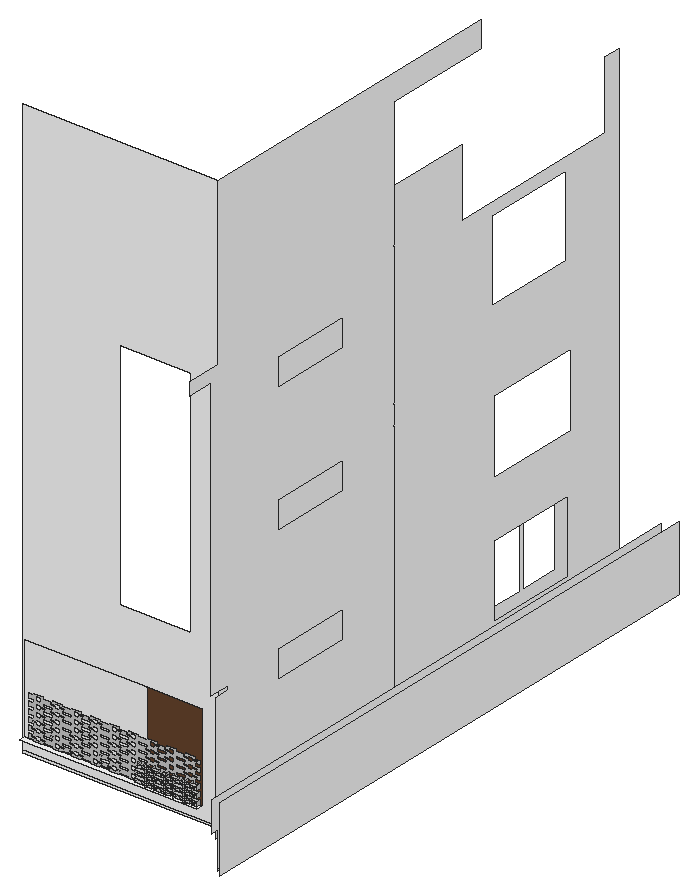
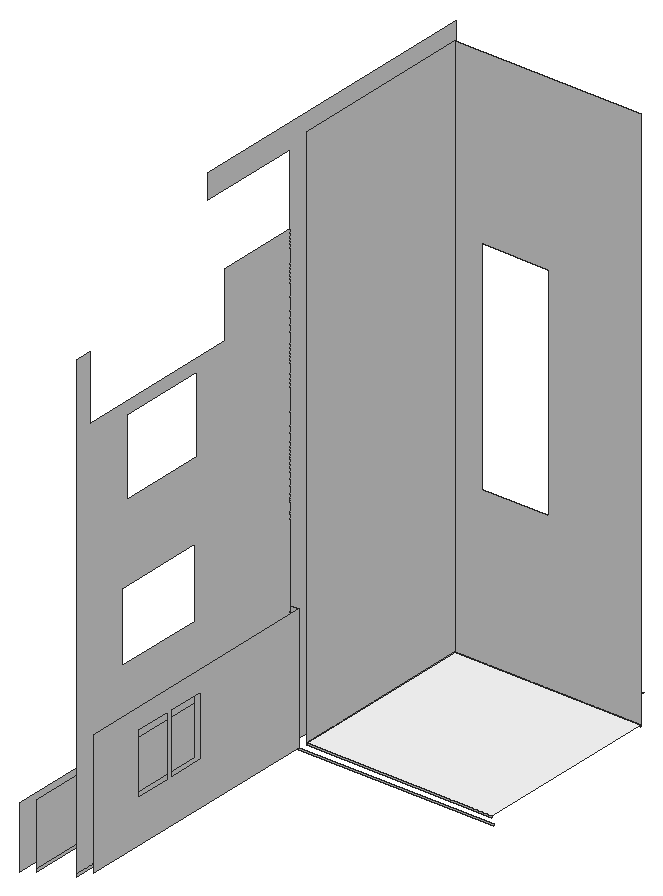
# SketchUp Ruby script. Lengths in inches.
U = 1.inch
M = Sketchup.active_model
def pt(a) = Geom::Point3d.new(a.map { |v| v * U })
def face(e, loops, mat)
  f = e.add_face(loops[0].map { |a| pt(a) })
  loops[1..].each { |l| e.add_face(l.map { |a| pt(a) }).erase! }
  f.material = f.back_material = mat if mat
  f
end
# faces: each face lists its corners as indices into pts; further lists are holes
def faces(e, pts, list, mat = nil) = list.each { |f| face(e, (f[0].is_a?(Array) ? f : [f]).map { |l| l.map { |i| pts[i] } }, mat) }
# xy, xz, yz: faces in a plane at the given z, y or x. An outline is a flat list of corners, or four numbers for a rectangle; further outlines are holes
def ring(l) = l.size == 4 ? [[l[0], l[1]], [l[2], l[1]], [l[2], l[3]], [l[0], l[3]]] : l.each_slice(2).to_a
def flat(e, list, mat, &to3) = list.each { |f| face(e, (f[0].is_a?(Array) ? f : [f]).map { |l| ring(l).map { |u, v| to3.(u, v) } }, mat) }
def xy(e, z, list, mat = nil) = flat(e, list, mat) { |x, y| [x, y, z] }
def xz(e, y, list, mat = nil) = flat(e, list, mat) { |x, z| [x, y, z] }
def yz(e, x, list, mat = nil) = flat(e, list, mat) { |y, z| [x, y, z] }
def lines(e, pts, list) = list.each { |a, b| e.add_line(pt(pts[a]), pt(pts[b])) }
# prism: a flat outline (further loops are holes) pulled along v
def prism(e, loops, v, mat = nil)
  f = face(e, loops, mat); d = Geom::Vector3d.new(v.map { |x| x * U })
  f.pushpull(f.normal.samedirection?(d) ? d.length : -d.length)
end
def box(e, o, s, mat = nil) = prism(e, [[o, [o[0] + s[0], o[1], o[2]], [o[0] + s[0], o[1] + s[1], o[2]], [o[0], o[1] + s[1], o[2]]]], [0, 0, s[2]], mat)
def at(x, y, z, deg = 0) = Geom::Transformation.translation(pt([x, y, z])) * Geom::Transformation.rotation(ORIGIN, Z_AXIS, deg.degrees)
def axes(o, x, y, z) = Geom::Transformation.new([*x, 0, *y, 0, *z, 0, *pt(o).to_a, 1])
def part(name) = M.definitions.add(name)
# library, detail: a bought-in or finely detailed component or shape, given as its bounding box
def library(name, o, s) = part(name).tap { |d| box(d.entities, o, s) }
def detail(e, o, s) = box(e.add_group.entities, o, s)
def put(e, d, t, mat = nil) = e.add_instance(d, t).tap { |i| i.material = mat if mat }
def group(e, t, mat = nil) = e.add_group.tap { |g| g.transformation = t; g.material = mat if mat }.entities
root = M.entities
M.materials.add("M00_Soft_Cloud").color = [255, 255, 255]
M.materials.add("Metal_Perforated_03_1K").color = [205, 205, 205]
M.materials.add("Wood_Veneer_15_1K1").color = [103, 69, 45]
xy(root,0,[[375,129,555,309]],"M00_Soft_Cloud")
xy(root,18,[[384,114,546,120]],"M00_Soft_Cloud")
xy(root,18,[[497.5,115.4375,505.72,119.17],[514.95,115.4375,523.18,119.17],[532.4,115.4375,540.63,119.17]],"Metal_Perforated_03_1K")
xy(root,19.23,[[499.55,115.4375,503.68,119.17],[517,115.4375,521.13,119.17],[534.45,115.4375,538.58,119.17]],"Metal_Perforated_03_1K")
xy(root,19.33,[[488.27,115.4375,497.5,119.17],[505.72,115.4375,514.95,119.17],[523.18,115.4375,532.4,119.17],[540.63,115.4375,545.24,119.17]],"Metal_Perforated_03_1K")
xy(root,20.57,[[494.94,115.4375,499.55,119.17],[503.68,115.4375,508.29,119.17],[512.39,115.4375,517,119.17],[521.13,115.4375,525.74,119.17],[529.84,115.4375,534.45,119.17],
  [538.58,115.4375,543.19,119.17]],"Metal_Perforated_03_1K")
xy(root,21.93,[[494.94,115.4375,499.55,119.17],[503.68,115.4375,508.29,119.17],[512.39,115.4375,517,119.17],[521.13,115.4375,525.74,119.17],[529.84,115.4375,534.45,119.17],
  [538.58,115.4375,543.19,119.17]],"Metal_Perforated_03_1K")
xy(root,23.16,[[488.27,115.4375,497.5,119.17],[505.72,115.4375,514.95,119.17],[523.18,115.4375,532.4,119.17],[540.63,115.4375,545.24,119.17]],"Metal_Perforated_03_1K")
xy(root,23.26,[[499.55,115.4375,503.68,119.17],[517,115.4375,521.13,119.17],[534.45,115.4375,538.58,119.17]],"Metal_Perforated_03_1K")
xy(root,25.73,[[499.55,115.4375,503.68,119.17],[517,115.4375,521.13,119.17],[534.45,115.4375,538.58,119.17]],"Metal_Perforated_03_1K")
xy(root,25.83,[[488.27,115.4375,497.5,119.17],[505.72,115.4375,514.95,119.17],[523.18,115.4375,532.4,119.17],[540.63,115.4375,545.24,119.17]],"Metal_Perforated_03_1K")
xy(root,27.06,[[494.94,115.4375,499.55,119.17],[503.68,115.4375,508.29,119.17],[512.39,115.4375,517,119.17],[521.13,115.4375,525.74,119.17],[529.84,115.4375,534.45,119.17],
  [538.58,115.4375,543.19,119.17]],"Metal_Perforated_03_1K")
xy(root,28.42,[[494.94,115.4375,499.55,119.17],[503.68,115.4375,508.29,119.17],[512.39,115.4375,517,119.17],[521.13,115.4375,525.74,119.17],[529.84,115.4375,534.45,119.17],
  [538.58,115.4375,543.19,119.17]],"Metal_Perforated_03_1K")
xy(root,29.65,[[488.27,115.4375,497.5,119.17],[505.72,115.4375,514.95,119.17],[523.18,115.4375,532.4,119.17],[540.63,115.4375,545.24,119.17]],"Metal_Perforated_03_1K")
xy(root,29.75,[[499.55,115.4375,503.68,119.17],[517,115.4375,521.13,119.17],[534.45,115.4375,538.58,119.17]],"Metal_Perforated_03_1K")
xy(root,32.22,[[499.55,115.4375,503.68,119.17],[517,115.4375,521.13,119.17],[534.45,115.4375,538.58,119.17]],"Metal_Perforated_03_1K")
xy(root,32.32,[[488.27,115.4375,497.5,119.17],[505.72,115.4375,514.95,119.17],[523.18,115.4375,532.4,119.17],[540.63,115.4375,545.24,119.17]],"Metal_Perforated_03_1K")
xy(root,33.55,[[494.94,115.4375,499.55,119.17],[503.68,115.4375,508.29,119.17],[512.39,115.4375,517,119.17],[521.13,115.4375,525.74,119.17],[529.84,115.4375,534.45,119.17],
  [538.58,115.4375,543.19,119.17]],"Metal_Perforated_03_1K")
xy(root,34.91,[[494.94,115.4375,499.55,119.17],[503.68,115.4375,508.29,119.17],[512.39,115.4375,517,119.17],[521.13,115.4375,525.74,119.17],[529.84,115.4375,534.45,119.17],
  [538.58,115.4375,543.19,119.17]],"Metal_Perforated_03_1K")
xz(root,119.17,[[[392.79,18,401.01,18,401.01,19.33,410.24,19.33,410.24,18,418.47,18,418.47,19.33,427.69,19.33,427.69,18,435.92,18,435.92,19.33,445.15,19.33,445.15,18,453.37,18,453.37,19.33,462.6,19.33,462.6,18,470.82,18,470.82,19.33,480.05,19.33,480.05,18,488.27,18,488.27,19.33,497.5,19.33,497.5,18,505.72,18,505.72,19.33,514.95,19.33,514.95,18,523.18,18,523.18,19.33,532.4,19.33,532.4,18,540.63,18,540.63,19.33,545.24,19.33,545.24,23.16,540.63,23.16,540.63,25.83,545.24,25.83,545.24,29.65,540.63,29.65,540.63,32.32,545.24,32.32,545.24,36.14,540.63,36.14,540.63,38.8125,545.24,38.8125,545.24,42.64,540.63,42.64,540.63,45.31,545.24,45.31,545.24,49.13,540.63,49.13,540.63,51.8,545.24,51.8,545.24,55.62,540.63,55.62,540.63,56.96,532.4,56.96,532.4,55.62,523.18,55.62,523.18,56.96,514.95,56.96,514.95,55.62,505.72,55.62,505.72,56.96,497.5,56.96,497.5,55.62,488.27,55.62,488.27,56.96,480.05,56.96,480.05,55.62,470.82,55.62,470.82,56.96,462.6,56.96,462.6,55.62,453.37,55.62,453.37,56.96,445.15,56.96,445.15,55.62,435.92,55.62,435.92,56.96,427.69,56.96,427.69,55.62,418.47,55.62,418.47,56.96,410.24,56.96,410.24,55.62,401.01,55.62,401.01,56.96,392.79,56.96,392.79,55.62,388.18,55.62,388.18,51.8,392.79,51.8,392.79,49.13,388.18,49.13,388.18,45.31,392.79,45.31,392.79,42.64,388.18,42.64,388.18,38.8125,392.79,38.8125,392.79,36.14,388.18,36.14,388.18,32.32,392.79,32.32,392.79,29.65,388.18,29.65,388.18,25.83,392.79,25.83,392.79,23.16,388.18,23.16,388.18,19.33,392.79,19.33],[464.65,51.7,464.65,53.03,460.03,53.03,460.03,54.39,464.65,54.39,464.65,55.72,468.77,55.72,468.77,54.39,473.39,54.39,473.39,53.03,468.77,53.03,468.77,51.7],[482.1,51.7,482.1,53.03,477.48,53.03,477.48,54.39,482.1,54.39,482.1,55.72,486.22,55.72,486.22,54.39,490.84,54.39,490.84,53.03,486.22,53.03,486.22,51.7],[464.65,25.73,464.65,27.06,460.03,27.06,460.03,28.42,464.65,28.42,464.65,29.75,468.77,29.75,468.77,28.42,473.39,28.42,473.39,27.06,468.77,27.06,468.77,25.73],[464.65,32.22,464.65,33.55,460.03,33.55,460.03,34.91,464.65,34.91,464.65,36.25,468.77,36.25,468.77,34.91,473.39,34.91,473.39,33.55,468.77,33.55,468.77,32.22],[464.65,19.23,464.65,20.57,460.03,20.57,460.03,21.93,464.65,21.93,464.65,23.26,468.77,23.26,468.77,21.93,473.39,21.93,473.39,20.57,468.77,20.57,468.77,19.23],[464.65,45.2,464.65,46.54,460.03,46.54,460.03,47.9,464.65,47.9,464.65,49.23,468.77,49.23,468.77,47.9,473.39,47.9,473.39,46.54,468.77,46.54,468.77,45.2],[482.1,25.73,482.1,27.06,477.48,27.06,477.48,28.42,482.1,28.42,482.1,29.75,486.22,29.75,486.22,28.42,490.84,28.42,490.84,27.06,486.22,27.06,486.22,25.73],[482.1,32.22,482.1,33.55,477.48,33.55,477.48,34.91,482.1,34.91,482.1,36.25,486.22,36.25,486.22,34.91,490.84,34.91,490.84,33.55,486.22,33.55,486.22,32.22],[482.1,19.23,482.1,20.57,477.48,20.57,477.48,21.93,482.1,21.93,482.1,23.26,486.22,23.26,486.22,21.93,490.84,21.93,490.84,20.57,486.22,20.57,486.22,19.23],[482.1,45.2,482.1,46.54,477.48,46.54,477.48,47.9,482.1,47.9,482.1,49.23,486.22,49.23,486.22,47.9,490.84,47.9,490.84,46.54,486.22,46.54,486.22,45.2],[464.65,38.71,464.65,40.05,460.03,40.05,460.03,41.4,464.65,41.4,464.65,42.74,468.77,42.74,468.77,41.4,473.39,41.4,473.39,40.05,468.77,40.05,468.77,38.71],[482.1,38.71,482.1,40.05,477.48,40.05,477.48,41.4,482.1,41.4,482.1,42.74,486.22,42.74,486.22,41.4,490.84,41.4,490.84,40.05,486.22,40.05,486.22,38.71],[394.84,51.7,394.84,53.03,390.22,53.03,390.22,54.39,394.84,54.39,394.84,55.72,398.97,55.72,398.97,54.39,403.58,54.39,403.58,53.03,398.97,53.03,398.97,51.7],[394.84,25.73,394.84,27.06,390.22,27.06,390.22,28.42,394.84,28.42,394.84,29.75,398.97,29.75,398.97,28.42,403.58,28.42,403.58,27.06,398.97,27.06,398.97,25.73],[394.84,19.23,394.84,20.57,390.22,20.57,390.22,21.93,394.84,21.93,394.84,23.26,398.97,23.26,398.97,21.93,403.58,21.93,403.58,20.57,398.97,20.57,398.97,19.23],[394.84,32.22,394.84,33.55,390.22,33.55,390.22,34.91,394.84,34.91,394.84,36.25,398.97,36.25,398.97,34.91,403.58,34.91,403.58,33.55,398.97,33.55,398.97,32.22],[394.84,45.2,394.84,46.54,390.22,46.54,390.22,47.9,394.84,47.9,394.84,49.23,398.97,49.23,398.97,47.9,403.58,47.9,403.58,46.54,398.97,46.54,398.97,45.2],[517,51.7,517,53.03,512.39,53.03,512.39,54.39,517,54.39,517,55.72,521.13,55.72,521.13,54.39,525.74,54.39,525.74,53.03,521.13,53.03,521.13,51.7],[517,25.73,517,27.06,512.39,27.06,512.39,28.42,517,28.42,517,29.75,521.13,29.75,521.13,28.42,525.74,28.42,525.74,27.06,521.13,27.06,521.13,25.73],[517,32.22,517,33.55,512.39,33.55,512.39,34.91,517,34.91,517,36.25,521.13,36.25,521.13,34.91,525.74,34.91,525.74,33.55,521.13,33.55,521.13,32.22],[517,19.23,517,20.57,512.39,20.57,512.39,21.93,517,21.93,517,23.26,521.13,23.26,521.13,21.93,525.74,21.93,525.74,20.57,521.13,20.57,521.13,19.23],[394.84,38.71,394.84,40.05,390.22,40.05,390.22,41.4,394.84,41.4,394.84,42.74,398.97,42.74,398.97,41.4,403.58,41.4,403.58,40.05,398.97,40.05,398.97,38.71],[517,45.2,517,46.54,512.39,46.54,512.39,47.9,517,47.9,517,49.23,521.13,49.23,521.13,47.9,525.74,47.9,525.74,46.54,521.13,46.54,521.13,45.2],[517,38.71,517,40.05,512.39,40.05,512.39,41.4,517,41.4,517,42.74,521.13,42.74,521.13,41.4,525.74,41.4,525.74,40.05,521.13,40.05,521.13,38.71],[412.29,51.7,412.29,53.03,407.68,53.03,407.68,54.39,412.29,54.39,412.29,55.72,416.42,55.72,416.42,54.39,421.03,54.39,421.03,53.03,416.42,53.03,416.42,51.7],[412.29,19.23,412.29,20.57,407.68,20.57,407.68,21.93,412.29,21.93,412.29,23.26,416.42,23.26,416.42,21.93,421.03,21.93,421.03,20.57,416.42,20.57,416.42,19.23],[429.74,51.7,429.74,53.03,425.13,53.03,425.13,54.39,429.74,54.39,429.74,55.72,433.87,55.72,433.87,54.39,438.48,54.39,438.48,53.03,433.87,53.03,433.87,51.7],[412.29,25.73,412.29,27.06,407.68,27.06,407.68,28.42,412.29,28.42,412.29,29.75,416.42,29.75,416.42,28.42,421.03,28.42,421.03,27.06,416.42,27.06,416.42,25.73],[412.29,32.22,412.29,33.55,407.68,33.55,407.68,34.91,412.29,34.91,412.29,36.25,416.42,36.25,416.42,34.91,421.03,34.91,421.03,33.55,416.42,33.55,416.42,32.22],[412.29,45.2,412.29,46.54,407.68,46.54,407.68,47.9,412.29,47.9,412.29,49.23,416.42,49.23,416.42,47.9,421.03,47.9,421.03,46.54,416.42,46.54,416.42,45.2],[429.74,32.22,429.74,33.55,425.13,33.55,425.13,34.91,429.74,34.91,429.74,36.25,433.87,36.25,433.87,34.91,438.48,34.91,438.48,33.55,433.87,33.55,433.87,32.22],[429.74,25.73,429.74,27.06,425.13,27.06,425.13,28.42,429.74,28.42,429.74,29.75,433.87,29.75,433.87,28.42,438.48,28.42,438.48,27.06,433.87,27.06,433.87,25.73],[429.74,19.23,429.74,20.57,425.13,20.57,425.13,21.93,429.74,21.93,429.74,23.26,433.87,23.26,433.87,21.93,438.48,21.93,438.48,20.57,433.87,20.57,433.87,19.23],[429.74,45.2,429.74,46.54,425.13,46.54,425.13,47.9,429.74,47.9,429.74,49.23,433.87,49.23,433.87,47.9,438.48,47.9,438.48,46.54,433.87,46.54,433.87,45.2],[534.45,51.7,534.45,53.03,529.84,53.03,529.84,54.39,534.45,54.39,534.45,55.72,538.58,55.72,538.58,54.39,543.19,54.39,543.19,53.03,538.58,53.03,538.58,51.7],[412.29,38.71,412.29,40.05,407.68,40.05,407.68,41.4,412.29,41.4,412.29,42.74,416.42,42.74,416.42,41.4,421.03,41.4,421.03,40.05,416.42,40.05,416.42,38.71],[534.45,25.73,534.45,27.06,529.84,27.06,529.84,28.42,534.45,28.42,534.45,29.75,538.58,29.75,538.58,28.42,543.19,28.42,543.19,27.06,538.58,27.06,538.58,25.73],[447.19,51.7,447.19,53.03,442.58,53.03,442.58,54.39,447.19,54.39,447.19,55.72,451.32,55.72,451.32,54.39,455.93,54.39,455.93,53.03,451.32,53.03,451.32,51.7],[534.45,32.22,534.45,33.55,529.84,33.55,529.84,34.91,534.45,34.91,534.45,36.25,538.58,36.25,538.58,34.91,543.19,34.91,543.19,33.55,538.58,33.55,538.58,32.22],[534.45,19.23,534.45,20.57,529.84,20.57,529.84,21.93,534.45,21.93,534.45,23.26,538.58,23.26,538.58,21.93,543.19,21.93,543.19,20.57,538.58,20.57,538.58,19.23],[429.74,38.71,429.74,40.05,425.13,40.05,425.13,41.4,429.74,41.4,429.74,42.74,433.87,42.74,433.87,41.4,438.48,41.4,438.48,40.05,433.87,40.05,433.87,38.71],[534.45,45.2,534.45,46.54,529.84,46.54,529.84,47.9,534.45,47.9,534.45,49.23,538.58,49.23,538.58,47.9,543.19,47.9,543.19,46.54,538.58,46.54,538.58,45.2],[447.19,25.73,447.19,27.06,442.58,27.06,442.58,28.42,447.19,28.42,447.19,29.75,451.32,29.75,451.32,28.42,455.93,28.42,455.93,27.06,451.32,27.06,451.32,25.73],[447.19,19.23,447.19,20.57,442.58,20.57,442.58,21.93,447.19,21.93,447.19,23.26,451.32,23.26,451.32,21.93,455.93,21.93,455.93,20.57,451.32,20.57,451.32,19.23],[447.19,32.22,447.19,33.55,442.58,33.55,442.58,34.91,447.19,34.91,447.19,36.25,451.32,36.25,451.32,34.91,455.93,34.91,455.93,33.55,451.32,33.55,451.32,32.22],[447.19,45.2,447.19,46.54,442.58,46.54,442.58,47.9,447.19,47.9,447.19,49.23,451.32,49.23,451.32,47.9,455.93,47.9,455.93,46.54,451.32,46.54,451.32,45.2],[534.45,38.71,534.45,40.05,529.84,40.05,529.84,41.4,534.45,41.4,534.45,42.74,538.58,42.74,538.58,41.4,543.19,41.4,543.19,40.05,538.58,40.05,538.58,38.71],[499.55,51.7,499.55,53.03,494.94,53.03,494.94,54.39,499.55,54.39,499.55,55.72,503.68,55.72,503.68,54.39,508.29,54.39,508.29,53.03,503.68,53.03,503.68,51.7],[447.19,38.71,447.19,40.05,442.58,40.05,442.58,41.4,447.19,41.4,447.19,42.74,451.32,42.74,451.32,41.4,455.93,41.4,455.93,40.05,451.32,40.05,451.32,38.71],[499.55,25.73,499.55,27.06,494.94,27.06,494.94,28.42,499.55,28.42,499.55,29.75,503.68,29.75,503.68,28.42,508.29,28.42,508.29,27.06,503.68,27.06,503.68,25.73],[499.55,19.23,499.55,20.57,494.94,20.57,494.94,21.93,499.55,21.93,499.55,23.26,503.68,23.26,503.68,21.93,508.29,21.93,508.29,20.57,503.68,20.57,503.68,19.23],[499.55,32.22,499.55,33.55,494.94,33.55,494.94,34.91,499.55,34.91,499.55,36.25,503.68,36.25,503.68,34.91,508.29,34.91,508.29,33.55,503.68,33.55,503.68,32.22],[499.55,45.2,499.55,46.54,494.94,46.54,494.94,47.9,499.55,47.9,499.55,49.23,503.68,49.23,503.68,47.9,508.29,47.9,508.29,46.54,503.68,46.54,503.68,45.2],[499.55,38.71,499.55,40.05,494.94,40.05,494.94,41.4,499.55,41.4,499.55,42.74,503.68,42.74,503.68,41.4,508.29,41.4,508.29,40.05,503.68,40.05,503.68,38.71],[418.47,36.14,427.69,38.8125],[470.82,36.14,480.05,38.8125],[418.47,42.64,427.69,45.31],[418.47,29.65,427.69,32.32],[470.82,42.64,480.05,45.31],[470.82,29.65,480.05,32.32],[418.47,23.16,427.69,25.83],[470.82,23.16,480.05,25.83],[418.47,49.13,427.69,51.8],[470.82,49.13,480.05,51.8],[488.27,36.14,497.5,38.8125],[488.27,42.64,497.5,45.31],[488.27,29.65,497.5,32.32],[488.27,23.16,497.5,25.83],[488.27,49.13,497.5,51.8],[453.37,36.14,462.6,38.8125],[453.37,29.65,462.6,32.32],[523.18,36.14,532.4,38.8125],[453.37,23.16,462.6,25.83],[523.18,42.64,532.4,45.31],[453.37,42.64,462.6,45.31],[523.18,29.65,532.4,32.32],[523.18,23.16,532.4,25.83],[453.37,49.13,462.6,51.8],[505.72,36.14,514.95,38.8125],[435.92,36.14,445.15,38.8125],[435.92,42.64,445.15,45.31],[523.18,49.13,532.4,51.8],[505.72,29.65,514.95,32.32],[435.92,29.65,445.15,32.32],[435.92,23.16,445.15,25.83],[505.72,23.16,514.95,25.83],[505.72,42.64,514.95,45.31],[505.72,49.13,514.95,51.8],[435.92,49.13,445.15,51.8],[401.01,36.14,410.24,38.8125],[401.01,29.65,410.24,32.32],[401.01,23.16,410.24,25.83],[401.01,42.64,410.24,45.31],[401.01,49.13,410.24,51.8]]],"Metal_Perforated_03_1K")
xz(root,120,[[384,18,495.39,98]],"M00_Soft_Cloud")
xz(root,120,[[495.39,18,546,98]],"Wood_Veneer_15_1K1")
xz(root,129,[[375,-1.88,555,0],[[375,0,555,531.06],[463.6,150.23,528.82,364.36]]],"M00_Soft_Cloud")
xz(root,309,[[375,-1.88,555,0]],"M00_Soft_Cloud")
xz(root,318,[[366,-1.88,555,0],[555,-1.88,564,0],[555,0,564,120]],"M00_Soft_Cloud")
yz(root,490.84,[[115.4375,27.06,119.17,28.42],[115.4375,33.55,119.17,34.91]],"Metal_Perforated_03_1K")
yz(root,494.94,[[115.4375,20.57,119.17,21.93],[115.4375,27.06,119.17,28.42],[115.4375,33.55,119.17,34.91]],"Metal_Perforated_03_1K")
yz(root,497.5,[[115.4375,18,119.17,19.33],[115.4375,23.16,119.17,25.83],[115.4375,29.65,119.17,32.32]],"Metal_Perforated_03_1K")
yz(root,499.55,[[115.4375,19.23,119.17,20.57],[115.4375,21.93,119.17,23.26],[115.4375,25.73,119.17,27.06],[115.4375,28.42,119.17,29.75],[115.4375,32.22,119.17,33.55],
  [115.4375,34.91,119.17,36.25]],"Metal_Perforated_03_1K")
yz(root,503.68,[[115.4375,19.23,119.17,20.57],[115.4375,21.93,119.17,23.26],[115.4375,25.73,119.17,27.06],[115.4375,28.42,119.17,29.75],[115.4375,32.22,119.17,33.55],
  [115.4375,34.91,119.17,36.25]],"Metal_Perforated_03_1K")
yz(root,505.72,[[115.4375,18,119.17,19.33],[115.4375,23.16,119.17,25.83],[115.4375,29.65,119.17,32.32]],"Metal_Perforated_03_1K")
yz(root,508.29,[[115.4375,20.57,119.17,21.93],[115.4375,27.06,119.17,28.42],[115.4375,33.55,119.17,34.91]],"Metal_Perforated_03_1K")
yz(root,512.39,[[115.4375,20.57,119.17,21.93],[115.4375,27.06,119.17,28.42],[115.4375,33.55,119.17,34.91]],"Metal_Perforated_03_1K")
yz(root,514.95,[[115.4375,18,119.17,19.33],[115.4375,23.16,119.17,25.83],[115.4375,29.65,119.17,32.32]],"Metal_Perforated_03_1K")
yz(root,517,[[115.4375,19.23,119.17,20.57],[115.4375,21.93,119.17,23.26],[115.4375,25.73,119.17,27.06],[115.4375,28.42,119.17,29.75],[115.4375,32.22,119.17,33.55],
  [115.4375,34.91,119.17,36.25]],"Metal_Perforated_03_1K")
yz(root,521.13,[[115.4375,19.23,119.17,20.57],[115.4375,21.93,119.17,23.26],[115.4375,25.73,119.17,27.06],[115.4375,28.42,119.17,29.75],[115.4375,32.22,119.17,33.55],
  [115.4375,34.91,119.17,36.25]],"Metal_Perforated_03_1K")
yz(root,523.18,[[115.4375,18,119.17,19.33],[115.4375,23.16,119.17,25.83],[115.4375,29.65,119.17,32.32]],"Metal_Perforated_03_1K")
yz(root,525.74,[[115.4375,20.57,119.17,21.93],[115.4375,27.06,119.17,28.42],[115.4375,33.55,119.17,34.91]],"Metal_Perforated_03_1K")
yz(root,529.84,[[115.4375,20.57,119.17,21.93],[115.4375,27.06,119.17,28.42],[115.4375,33.55,119.17,34.91]],"Metal_Perforated_03_1K")
yz(root,532.4,[[115.4375,18,119.17,19.33],[115.4375,23.16,119.17,25.83],[115.4375,29.65,119.17,32.32]],"Metal_Perforated_03_1K")
yz(root,534.45,[[115.4375,19.23,119.17,20.57],[115.4375,21.93,119.17,23.26],[115.4375,25.73,119.17,27.06],[115.4375,28.42,119.17,29.75],[115.4375,32.22,119.17,33.55],
  [115.4375,34.91,119.17,36.25]],"Metal_Perforated_03_1K")
yz(root,538.58,[[115.4375,19.23,119.17,20.57],[115.4375,21.93,119.17,23.26],[115.4375,25.73,119.17,27.06],[115.4375,28.42,119.17,29.75],[115.4375,32.22,119.17,33.55],
  [115.4375,34.91,119.17,36.25]],"Metal_Perforated_03_1K")
yz(root,540.63,[[115.4375,18,119.17,19.33],[115.4375,23.16,119.17,25.83],[115.4375,29.65,119.17,32.32]],"Metal_Perforated_03_1K")
yz(root,543.19,[[115.4375,20.57,119.17,21.93],[115.4375,27.06,119.17,28.42],[115.4375,33.55,119.17,34.91]],"Metal_Perforated_03_1K")
yz(root,545.24,[[115.4375,19.33,119.17,23.16],[115.4375,25.83,119.17,29.65],[115.4375,32.32,119.17,36.14]],"Metal_Perforated_03_1K")
yz(root,555,[[129,-1.88,309,0],[129,0,309,531.06],[[318,0,567,120],[477.4,42.1,513.74,100.83],[437.07,42.1,473.4,100.83]]],"M00_Soft_Cloud")
yz(root,564,[[318,-1.88,576,0],[[114,0,318,0,318,516.24,417.73,516.24,417.73,540.06,116.39,540.06,116.39,388.7,84.01,388.7,84.01,377.4375,108.01,377.4375,108.01,119.96,128.03,119.96,128.03,116,114,116],[184.64,99.76,259.82,125.08],[184.64,222.33,259.82,247.65],[184.64,339.72,259.82,365.04]],[[318,0,576,0,576,447.06,560.69,447.06,560.69,384.3,396.17,384.3,396.17,447.06,318,447.06],[430.94,298.875,515.79,372.92],[433.07,156.7,521.56,224.13],[433.07,38.1,517.74,104.83]]],"M00_Soft_Cloud")
yz(root,592.34,[[80.34,-1.88,589.09,0],[80.34,0,80.34,31.95,73.42,31.95,73.42,60,589.09,60,589.09,0]],"M00_Soft_Cloud")
yz(root,600,[[73.42,0,600,60]],"M00_Soft_Cloud")
